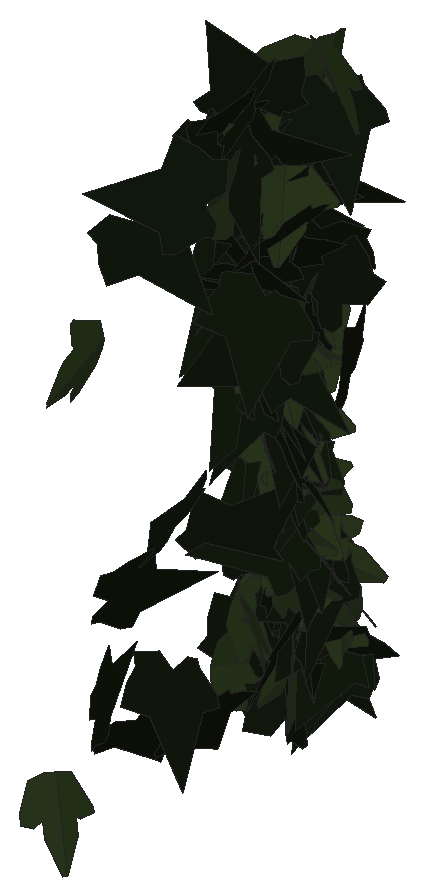
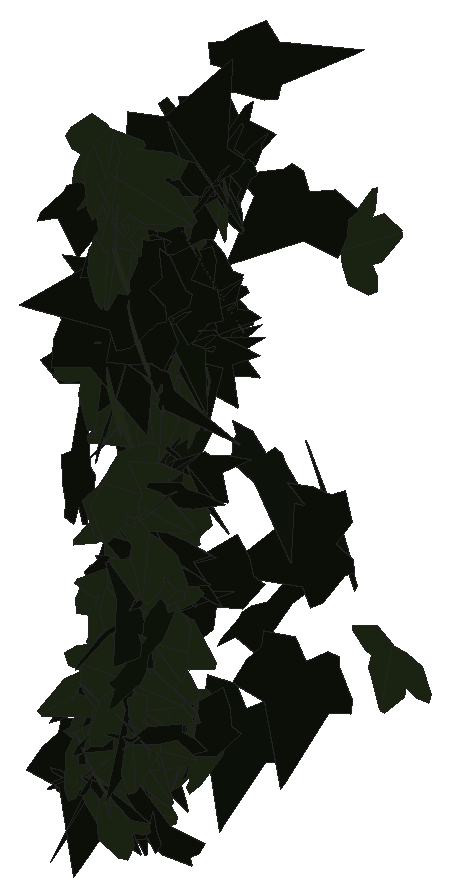
# SketchUp Ruby script. Lengths in inches.
U = 1.inch
M = Sketchup.active_model
def pt(a) = Geom::Point3d.new(a.map { |v| v * U })
def face(e, loops, mat)
  f = e.add_face(loops[0].map { |a| pt(a) })
  loops[1..].each { |l| e.add_face(l.map { |a| pt(a) }).erase! }
  f.material = f.back_material = mat if mat
  f
end
# faces: each face lists its corners as indices into pts; further lists are holes
def faces(e, pts, list, mat = nil) = list.each { |f| face(e, (f[0].is_a?(Array) ? f : [f]).map { |l| l.map { |i| pts[i] } }, mat) }
# xy, xz, yz: faces in a plane at the given z, y or x. An outline is a flat list of corners, or four numbers for a rectangle; further outlines are holes
def ring(l) = l.size == 4 ? [[l[0], l[1]], [l[2], l[1]], [l[2], l[3]], [l[0], l[3]]] : l.each_slice(2).to_a
def flat(e, list, mat, &to3) = list.each { |f| face(e, (f[0].is_a?(Array) ? f : [f]).map { |l| ring(l).map { |u, v| to3.(u, v) } }, mat) }
def xy(e, z, list, mat = nil) = flat(e, list, mat) { |x, y| [x, y, z] }
def xz(e, y, list, mat = nil) = flat(e, list, mat) { |x, z| [x, y, z] }
def yz(e, x, list, mat = nil) = flat(e, list, mat) { |y, z| [x, y, z] }
def lines(e, pts, list) = list.each { |a, b| e.add_line(pt(pts[a]), pt(pts[b])) }
# prism: a flat outline (further loops are holes) pulled along v
def prism(e, loops, v, mat = nil)
  f = face(e, loops, mat); d = Geom::Vector3d.new(v.map { |x| x * U })
  f.pushpull(f.normal.samedirection?(d) ? d.length : -d.length)
end
def box(e, o, s, mat = nil) = prism(e, [[o, [o[0] + s[0], o[1], o[2]], [o[0] + s[0], o[1] + s[1], o[2]], [o[0], o[1] + s[1], o[2]]]], [0, 0, s[2]], mat)
def at(x, y, z, deg = 0) = Geom::Transformation.translation(pt([x, y, z])) * Geom::Transformation.rotation(ORIGIN, Z_AXIS, deg.degrees)
def axes(o, x, y, z) = Geom::Transformation.new([*x, 0, *y, 0, *z, 0, *pt(o).to_a, 1])
def part(name) = M.definitions.add(name)
# library, detail: a bought-in or finely detailed component or shape, given as its bounding box
def library(name, o, s) = part(name).tap { |d| box(d.entities, o, s) }
def detail(e, o, s) = box(e.add_group.entities, o, s)
def put(e, d, t, mat = nil) = e.add_instance(d, t).tap { |i| i.material = mat if mat }
def group(e, t, mat = nil) = e.add_group.tap { |g| g.transformation = t; g.material = mat if mat }.entities
root = M.entities
M.materials.add("efeu1").color = [18, 25, 13]
M.materials.add("efeu2").color = [43, 57, 29]
c1 = part("ivyleaf_10")
p = [[0,0.5,-0.03],[-0.0625,2.02,-0.43],[-0.19,2.01,-0.46],[-0.54,1.05,-0.29],[-0.52,0.625,-0.18],[-0.83,0.76,-0.28],
  [-1.16,0.64,-0.33],[-1.15,0.33,-0.24],[-0.77,-0.39,0.02],[-0.3,-0.51,0.16],[0.04,-0.48,0.23],[-0.02,2.01,-0.4375],
  [-0.06,2.01,-0.43],[0.04,-0.49,0.23],[0.67,-0.49,0.14],[1.38,0.36,-0.2],[1.375,0.51,-0.24],[0.81,0.65,-0.19],
  [0.62,0.59,-0.15],[0.6,1.09,-0.28],[0.5,1.23,-0.31]]
faces(c1.entities,p,[[0,1,2,3,4,5,6,7,8,9,10],[11,12,0,13,14,15,16,17,18,19,20]],"efeu2")
c2 = part("ivyleaf_9")
p = [[1.54,2.16,1.25],[1.36,2.04,1.19],[-0.21,0.99,0.68],[-0.71,1.11,0.82],[-0.85,0.86,0.67],[-0.8,0.17,0.21],
  [-0.9,-0.01,0.1],[-0.67,-0.16,-0.02],[-0.08,-0.08,-0.05],[-0.03,-0.6,-0.4],[0.65,-0.88,-0.66],[0.83,-0.6,-0.49],
  [1.29,-0.42,-0.43],[1.8125,-0.07,-0.26],[1.21,0.44,0.15]]
faces(c2.entities,p,[[0,1,2,3,4,5,6,7,8,9,10,11,12,13,14]],"efeu1")
put(root,c1,axes([53.47,219.33,214.4],[0.45704,-0.01412,0.20227],[0.20232,-0.00106,-0.45724],[0.01334,0.4998,0.00475]))
put(root,c2,axes([54,219.53,215.61],[-0.09301,0.33525,0.35911],[0.09611,-0.34601,0.34791],[0.48178,0.13374,-0.00008]))
put(root,c1,axes([53.34,220.18,220.24],[0.05439,-0.10599,0.4856],[0.16699,-0.4562,-0.11828],[0.46814,0.17505,-0.01423]))
put(root,c2,axes([54.5625,220.84,222.49],[-0.22978,-0.0549,0.44067],[-0.41817,-0.14023,-0.23552],[0.14945,-0.47678,0.01853]))
put(root,c2,axes([54.08,220.91,215.59],[0.02323,-0.49581,-0.06029],[-0.00815,0.05997,-0.49632],[0.49939,0.02404,-0.0053]))
put(root,c2,axes([53.34,220.66,216.53],[0.2112,0.19575,0.40875],[0.30889,0.26781,-0.28786],[-0.33163,0.37411,-0.00781]))
put(root,c2,axes([53.63,220.79,214.85],[0.15717,0.47438,-0.01634],[-0.00665,-0.01501,-0.49973],[-0.47461,0.1573,0.00159]))
put(root,c2,axes([53.98,221.06,217.62],[-0.15319,0.43734,0.18779],[-0.08974,0.1672,-0.46259],[-0.46742,-0.17543,0.02727]))
put(root,c2,axes([53.2,221.3,221.49],[-0.08116,-0.15363,-0.46884],[0.22372,0.41202,-0.17374],[0.43973,-0.23798,0.00186]))
put(root,c2,axes([53.83,221.66,214.54],[0.0958,0.48707,0.05985],[0.0154,0.05797,-0.49639],[-0.49049,0.09695,-0.00389]))
put(root,c2,axes([53.6,222.34,222.27],[0.05873,-0.13634,-0.47745],[0.3246,-0.35328,0.14081],[-0.37575,-0.3265,0.04702]))
put(root,c2,axes([54.29,222.45,221.14],[-0.33156,0.20634,-0.31223],[0.18957,-0.26708,-0.3778],[-0.32269,-0.36891,0.09888]))
put(root,c2,axes([53.94,222.71,219.47],[-0.13657,-0.25069,0.41049],[-0.18242,-0.36785,-0.28533],[0.44506,-0.22769,0.00901]))
put(root,c2,axes([54.14,222.63,220.18],[-0.22139,-0.43521,-0.10761],[0.07488,0.08244,-0.48744],[0.44202,-0.23194,0.02868]))
put(root,c2,axes([53.73,222.52,222.24],[-0.23742,-0.09868,-0.42883],[0.39803,0.15961,-0.2571],[0.18763,-0.46345,0.00277]))
put(root,c1,axes([53.88,222.09,221.6875],[0.06079,0.01229,0.49614],[-0.22717,0.4451,0.01681],[-0.44125,-0.22746,0.0597]))
put(root,c2,axes([53.34,222.49,222.29],[0.21797,-0.39358,-0.21814],[-0.10411,0.1917,-0.4499],[0.43778,0.24155,0.00162]))
put(root,c1,axes([53.55,222.63,222.17],[-0.37502,0.1499,-0.29477],[0.20132,-0.2501,-0.38331],[-0.26235,-0.40618,0.12723]))
put(root,c2,axes([53.55,223.05,220.01],[-0.32264,-0.36441,0.11448],[-0.03267,-0.12297,-0.48354],[0.38057,-0.3195,0.05554]))
put(root,c2,axes([53.42,222.8,220.5],[0.26216,-0.19668,0.37761],[0.32785,-0.18967,-0.32641],[0.27163,0.41874,0.02952]))
put(root,c2,axes([53.59,222.54,216.48],[-0.09428,-0.05385,0.48807],[0.4814,0.08782,0.10268],[-0.09679,0.48927,0.03528]))
put(root,c2,axes([53.51,222.32,222.43],[0.21033,0.24671,0.38065],[0.16327,0.35028,-0.31724],[-0.42321,0.25775,0.06679]))
put(root,c2,axes([53.9,222.69,222.86],[-0.35354,0.35307,-0.01877],[0.01329,-0.01326,-0.49965],[-0.35332,-0.35379,0]))
put(root,c2,axes([53.8125,222.64,220.5],[0.11834,0.44295,-0.19949],[-0.10328,-0.17769,-0.45581],[-0.47469,0.14909,0.04944]))
put(root,c1,axes([53.52,222.89,219.55],[-0.23828,0.28258,-0.33671],[0.22949,-0.24669,-0.36943],[-0.37491,-0.3306,-0.01214]))
put(root,c2,axes([53.5,223.01,220.34],[-0.10372,-0.4838,-0.07198],[0.01572,0.07024,-0.49479],[0.48887,-0.1049,0.00064]))
put(root,c2,axes([54.39,222.55,221.22],[0.03375,0.49552,0.05766],[-0.01993,0.05909,-0.4961],[-0.49846,0.03119,0.02374]))
put(root,c2,axes([53.62,222.96,221.45],[-0.44295,0.1099,-0.20424],[0.1989,-0.04646,-0.45638],[-0.11929,-0.48555,-0.00256]))
put(root,c2,axes([53.42,223.02,220.63],[0.05885,-0.4881,-0.09108],[0.02288,0.09429,-0.4905],[0.496,0.05356,0.03344]))
put(root,c2,axes([53.58,223.13,220.15],[-0.38781,-0.31167,-0.04966],[0.03391,0.03707,-0.49747],[0.31378,-0.38921,-0.00761]))
put(root,c2,axes([53.8,223.11,218.66],[-0.4671,0.01305,-0.17791],[0.17691,-0.02998,-0.46669],[-0.02285,-0.49893,0.02339]))
put(root,c1,axes([54.19,222.98,221.66],[0.28978,0.40413,-0.05207],[-0.03386,-0.03979,-0.49726],[-0.40606,0.29172,0.00431]))
put(root,c2,axes([53.56,223.29,217.78],[0.06969,-0.17383,0.4636],[0.15332,-0.43758,-0.18712],[0.47078,0.16824,-0.00769]))
put(root,c2,axes([54.12,223.34,216.48],[-0.29618,-0.10764,0.38818],[-0.30507,-0.25472,-0.3034],[0.26308,-0.41657,0.08521]))
put(root,c2,axes([54.16,222.85,219.15],[-0.47438,0.1547,0.03207],[0.02004,-0.04176,0.49785],[0.15671,0.47363,0.03342]))
put(root,c2,axes([53.6,223.17,222.54],[0.26503,0.10546,0.41065],[-0.41185,-0.05096,0.27889],[0.10068,-0.48609,0.05985]))
put(root,c2,axes([53.48,222.91,222],[0.27008,-0.00035,0.42078],[0.42073,0.00781,-0.27005],[-0.00638,0.49994,0.00451]))
put(root,c2,axes([54.07,222.95,219.33],[0.30816,-0.30373,-0.25056],[-0.07503,0.26705,-0.416],[0.38653,0.29399,0.11902]))
put(root,c1,axes([54.02,223.37,214.64],[-0.09182,0.20633,-0.44609],[0.15642,-0.41794,-0.22551],[-0.46594,-0.18097,0.0122]))
put(root,c2,axes([53.48,223.42,218.65],[-0.2953,-0.40096,0.04504],[0.01521,-0.06684,-0.49528],[0.40319,-0.29115,0.05167]))
put(root,c1,axes([53.5,222.73,214.73],[-0.02372,0.1363,0.48048],[-0.07574,0.47448,-0.13834],[-0.49366,-0.07935,-0.00186]))
put(root,c2,axes([53.83,223.33,217.62],[0.01448,-0.00098,0.49979],[0.2449,-0.43584,-0.00795],[0.43568,0.24503,-0.01214]))
put(root,c1,axes([53.95,223.0625,219.15],[0.40735,0.24659,0.15252],[0.10752,0.1158,-0.47437],[-0.26927,0.41927,0.04131]))
put(root,c2,axes([53.79,223.22,218.59],[0.33112,-0.37195,0.04491],[0.03145,-0.03213,-0.49797],[0.37333,0.3326,0.00212]))
put(root,c1,axes([53.91,223.09,219.21],[0.47663,0.06535,0.13621],[0.11409,0.13979,-0.46631],[-0.09903,0.47559,0.11834]))
put(root,c1,axes([53.64,223.08,220.07],[-0.22078,0.44861,0.00311],[-0.00355,0.00172,-0.49998],[-0.4486,-0.22079,0.00243]))
put(root,c1,axes([53.85,223.1,219.72],[-0.02069,-0.46548,-0.1814],[-0.009,0.18187,-0.46566],[0.49949,-0.016,-0.0159]))
put(root,c2,axes([53.59,223.19,220.75],[0.34192,0.35436,0.08673],[-0.06353,-0.05922,0.4924],[0.35924,-0.34774,0.00452]))
put(root,c1,axes([53.48,222.88,222.16],[-0.05785,-0.07101,-0.49154],[0.2676,0.41242,-0.09108],[0.41838,-0.27361,-0.00972]))
put(root,c1,axes([53.52,223.11,215.36],[-0.39141,0.30174,0.07581],[-0.06203,0.0437,-0.49421],[-0.30488,-0.39628,0.00323]))
put(root,c1,axes([53.97,223.28,217.81],[0.4933,0.06307,-0.05176],[-0.05207,-0.00087,-0.49728],[-0.06281,0.49601,0.00571]))
put(root,c2,axes([53.71,223.08,220.75],[-0.20825,0.45121,0.05513],[-0.00999,0.05608,-0.49674],[-0.45446,-0.208,-0.01435]))
put(root,c2,axes([53.82,223.58,218.29],[-0.00935,-0.49417,0.07558],[-0.01528,-0.07527,-0.49407],[0.49968,-0.01155,-0.0137]))
put(root,c1,axes([53.79,223.01,219.11],[0.12164,-0.01465,0.48476],[0.22688,0.44343,-0.04353],[-0.42864,0.23055,0.11452]))
put(root,c1,axes([53.52,223.09,215.37],[-0.02719,0.44028,0.2354],[-0.01072,0.23518,-0.44111],[-0.49915,-0.02903,-0.00335]))
put(root,c2,axes([53.47,223.12,214.79],[-0.16113,-0.08895,0.46489],[0.41974,0.20013,0.18377],[-0.21877,0.44949,0.01018]))
put(root,c2,axes([54.05,223.43,215.28],[-0.27229,0.31633,-0.27531],[0.17829,-0.20979,-0.41737],[-0.37957,-0.32546,0.00145]))
put(root,c2,axes([53.95,223.25,217.97],[0.39999,-0.20776,-0.21644],[-0.19569,0.09275,-0.45067],[0.22741,0.44523,-0.00711]))
put(root,c1,axes([53.75,223.33,215.83],[-0.46901,0.03674,0.16936],[-0.17002,-0.00298,-0.47019],[-0.03354,-0.49864,0.01529]))
put(root,c1,axes([53.96,223.71,217.04],[-0.09442,-0.34082,0.35345],[0.08265,-0.36582,-0.33067],[0.484,-0.00402,0.12542]))
put(root,c2,axes([53.91,223.1,220.57],[0.33088,0.37219,0.04468],[0.00446,0.05568,-0.49687],[-0.37483,0.32921,0.03353]))
put(root,c2,axes([53.76,223.64,217.76],[-0.47605,-0.15276,-0.00653],[0.00646,0.00124,-0.49996],[0.15276,-0.47609,0.0008]))
put(root,c2,axes([54.04,223.82,221.79],[-0.02184,-0.10626,-0.48809],[0.1885,-0.45419,0.09044],[-0.46259,-0.18006,0.0599]))
put(root,c2,axes([53.79,223.67,217.68],[-0.40296,-0.29036,-0.05757],[0.04841,0.03128,-0.49667],[0.29203,-0.40584,0.0029]))
put(root,c1,axes([53.91,223.53,216.5625],[0.4134,0.24502,-0.13806],[-0.12504,-0.05974,-0.48041],[-0.25192,0.43173,0.01189]))
put(root,c2,axes([53.76,223.59,213.86],[-0.06694,0.17325,0.46422],[0.19852,-0.41982,0.18531],[0.45399,0.20913,-0.01259]))
put(root,c2,axes([53.26,223.55,218.81],[0.314,-0.38533,0.0541],[0.09573,0.00912,-0.49067],[0.37715,0.31849,0.0795]))
put(root,c2,axes([53.46,223.19,221.08],[0.0781,0.138,-0.47419],[0.16613,0.44477,0.15679],[0.46508,-0.18204,0.02362]))
put(root,c2,axes([53.96,223.81,216.3],[0.02001,-0.46268,0.18848],[0.05368,-0.18554,-0.46119],[0.49671,0.03869,0.04225]))
put(root,c1,axes([53.75,223.6,217.04],[0.24291,0.34652,0.2663],[-0.15055,-0.21968,0.42318],[0.41028,-0.28577,-0.00239]))
put(root,c2,axes([53.8,223.75,217.43],[-0.33401,-0.34396,-0.14188],[0.13652,0.06407,-0.47672],[0.34613,-0.35719,0.05111]))
put(root,c1,axes([53.49,223.46,216.34],[-0.00129,-0.06489,0.49577],[0.46553,0.18072,0.02487],[-0.18242,0.46166,0.05995]))
put(root,c1,axes([53.6,223.5,216.46],[-0.38706,-0.30517,-0.08401],[0.06762,0.04992,-0.49288],[0.30921,-0.39291,0.00262]))
put(root,c2,axes([53.89,223.64,219.86],[-0.43694,0.08429,0.22799],[-0.22302,0.04748,-0.44498],[-0.09666,-0.49055,-0.00389]))
put(root,c1,axes([53.99,223.6,221],[0.30226,-0.38995,-0.08109],[-0.05233,0.06203,-0.49337],[0.39484,0.30674,-0.00332]))
put(root,c1,axes([54.07,223.58,217.09],[-0.4293,-0.24454,0.07683],[-0.06707,-0.03747,-0.49406],[0.24739,-0.43451,-0.00063]))
put(root,c1,axes([53.96,223.63,218.04],[0.20228,0.45403,-0.05425],[-0.00769,-0.05593,-0.4968],[-0.45719,0.20182,-0.01565]))
put(root,c1,axes([53.68,223.68,215.62],[0.45745,0.1948,-0.05283],[-0.04901,-0.01976,-0.4972],[-0.1958,0.46007,0.00102]))
put(root,c1,axes([53.62,223.89,220.83],[0.24918,-0.35435,0.2497],[0.14397,-0.20402,-0.43319],[0.40888,0.28778,0.00036]))
put(root,c2,axes([53.88,223.89,216.71],[0.08142,-0.4927,0.02484],[0.00457,-0.02442,-0.49938],[0.49331,0.08154,0.00053]))
put(root,c2,axes([54.37,223.83,219.74],[0.04772,0.02256,0.49721],[-0.49708,-0.02318,0.04876],[0.02525,-0.49895,0.02022]))
put(root,c2,axes([53.93,224.09,219.37],[-0.01902,-0.11465,0.48631],[0.0133,-0.4866,-0.1142],[0.49946,0.00859,0.02156]))
put(root,c1,axes([53.97,223.84,219.82],[0.217,-0.44756,0.05099],[0.01887,-0.04752,-0.49738],[0.45006,0.21779,-0.00373]))
put(root,c2,axes([53.41,223.99,218.65],[-0.37258,-0.32539,-0.07284],[0.09743,-0.00178,-0.49041],[0.31889,-0.37963,0.06474]))
put(root,c2,axes([54.17,224.11,214.75],[-0.23354,-0.42315,0.12807],[0.06724,-0.17715,-0.46271],[0.43696,-0.1989,0.13965]))
put(root,c1,axes([53.2,223.58,218.39],[0.1673,0.11037,0.45807],[0.37027,0.26982,-0.20024],[-0.29139,0.40622,0.00855]))
put(root,c2,axes([53.83,224.15,215.03],[-0.176,-0.38646,0.26396],[0.03098,-0.29101,-0.4054],[0.46697,-0.12635,0.12638]))
put(root,c2,axes([53.74,223.59,213.79],[-0.47434,0.07747,0.13785],[0.13626,-0.02089,0.48062],[0.08022,0.49352,-0.0013]))
put(root,c1,axes([53.89,223.59,217.09],[0.1902,0.39099,0.24689],[0.11956,0.2163,-0.43465],[-0.44669,0.22438,-0.01121]))
put(root,c2,axes([53.89,223.71,216.26],[0.47262,-0.16139,-0.02422],[-0.02228,0.00969,-0.49941],[0.16167,0.47314,0.00197]))
put(root,c2,axes([54.13,223.77,220.65],[0.17111,0.31482,-0.34872],[-0.16789,-0.30565,-0.35832],[-0.43879,0.23972,0.00111]))
put(root,c1,axes([53.69,224.17,214.44],[-0.02126,-0.21802,0.44946],[0.03297,-0.4495,-0.21648],[0.49846,0.02044,0.03349]))
put(root,c1,axes([54.09,223.88,220.06],[-0.46112,-0.17205,-0.08816],[0.13862,-0.13535,-0.46094],[0.13475,-0.44953,0.17252]))
put(root,c1,axes([54.01,223.87,215.07],[0.47403,0.14284,0.06994],[0.06483,0.02725,-0.49503],[-0.14524,0.47839,0.00731]))
put(root,c2,axes([53.71,223.96,215.55],[0.02749,-0.46616,-0.17873],[-0.01944,0.17786,-0.46689],[0.49887,0.03262,-0.00834]))
put(root,c2,axes([53.3,223.82,220.96],[0.3444,0.14634,-0.33162],[0.27851,0.18594,0.37129],[0.23199,-0.44047,0.04656]))
put(root,c2,axes([53.96,224.11,215.66],[-0.33255,-0.18396,-0.32491],[0.35593,-0.02477,-0.35028],[0.11278,-0.46427,0.14743]))
put(root,c1,axes([53.62,224.08,222.74],[0.23023,0.25014,-0.36664],[-0.30328,-0.21291,-0.33569],[-0.32406,0.37696,0.05369]))
put(root,c2,axes([54.14,224.03,222.45],[-0.06025,-0.46037,-0.18556],[0.02293,0.18414,-0.46429],[0.49583,-0.06445,-0.00107]))
put(root,c1,axes([53.65,224.21,221.91],[0.1259,-0.11619,0.46973],[0.36726,-0.2931,-0.17093],[0.31508,0.38806,0.01154]))
put(root,c2,axes([53.61,223.83,215.69],[-0.08513,-0.15935,-0.46622],[0.20959,0.41647,-0.18062],[0.4459,-0.22619,-0.00411]))
put(root,c2,axes([53.72,223.78,217.08],[0.32727,-0.20255,-0.31916],[-0.22006,0.24117,-0.3787],[0.30736,0.38834,0.06871]))
put(root,c1,axes([53.99,223.89,215.4],[-0.49385,0.05823,0.05217],[-0.05199,0.00456,-0.49727],[-0.05839,-0.49658,0.00155]))
put(root,c2,axes([53.63,223.65,215.79],[0.04009,-0.04346,-0.49649],[-0.35049,0.35166,-0.05908],[0.35433,0.35277,-0.00227]))
put(root,c1,axes([53.81,224,215.33],[-0.32216,0.00045,0.38238],[-0.37171,-0.11764,-0.31303],[0.08969,-0.48596,0.07613]))
put(root,c2,axes([54.05,223.83,214.84],[0.26841,-0.24831,-0.34102],[-0.21332,0.26882,-0.36364],[0.36394,0.3407,0.03837]))
put(root,c2,axes([53.31,224.14,216.58],[0.28842,-0.37391,0.16433],[0.11115,-0.12173,-0.47205],[0.39302,0.30882,0.0129]))
put(root,c2,axes([54.17,224.21,214.57],[-0.45446,-0.14732,-0.14751],[0.15384,0.00178,-0.47574],[0.14069,-0.4778,0.04371]))
put(root,c2,axes([53.58,223.83,221.21],[0.36435,0.04864,0.33894],[0.33609,0.04385,-0.36759],[-0.06548,0.49569,-0.00074]))
put(root,c2,axes([53.43,224.2,215.43],[-0.21275,-0.42272,-0.16138],[0.09,0.13523,-0.47288],[0.44344,-0.23026,0.01855]))
put(root,c1,axes([54.07,224.01,222.99],[-0.41773,0.23003,-0.15028],[0.13552,-0.0654,-0.47682],[-0.23902,-0.4391,-0.00771]))
put(root,c1,axes([53.875,224.31,214.76],[0.01679,-0.16418,-0.47198],[0.30649,-0.36961,0.13947],[-0.39469,-0.29399,0.08823]))
put(root,c2,axes([54.17,223.85,214.86],[0.3292,0.34769,-0.14402],[-0.10536,-0.09854,-0.47874],[-0.36128,0.34555,0.00839]))
put(root,c1,axes([53.23,224.125,218.07],[0.46052,-0.06605,0.1832],[0.18324,-0.01225,-0.46505],[0.06592,0.49547,0.01292]))
put(root,c1,axes([53.73,224.34,221.91],[0.03114,-0.39178,0.30909],[0.11748,-0.29523,-0.38605],[0.485,0.09667,0.07367]))
put(root,c1,axes([53.87,224.22,222.95],[0.05494,-0.4794,0.13099],[0.0367,-0.12752,-0.48207],[0.49562,0.06259,0.02118]))
put(root,c1,axes([53.93,224.1,216.16],[0.10835,0.06209,-0.48416],[-0.48811,0.01604,-0.10718],[0.00223,0.49587,0.06409]))
put(root,c2,axes([53.8,223.68,216.83],[-0.02205,0.27078,0.41975],[-0.01351,0.41969,-0.27144],[-0.49933,-0.02331,-0.0112]))
put(root,c1,axes([53.68,224.33,215.41],[-0.06781,-0.09241,0.48668],[-0.30402,-0.38007,-0.11453],[0.39112,-0.31146,-0.00464]))
put(root,c1,axes([53.52,224.36,218.86],[0.07869,0.24429,-0.42911],[-0.25859,-0.34978,-0.24655],[-0.42064,0.26073,0.07129]))
put(root,c2,axes([54.16,224.31,218.43],[0.02272,0.2041,0.45588],[-0.06472,-0.4513,0.20527],[0.49527,-0.06834,0.00591]))
put(root,c1,axes([54.09,224.21,215.09],[-0.01631,-0.49515,0.06751],[0.03384,-0.06849,-0.49413],[0.49859,-0.01155,0.03575]))
put(root,c1,axes([53.89,223.9375,216.06],[-0.23222,-0.14412,-0.41869],[0.37823,0.18127,-0.27218],[0.23024,-0.44314,0.02483]))
put(root,c1,axes([53.79,223.95,222.08],[0.03701,-0.41224,-0.28052],[-0.00076,0.28124,-0.4134],[0.49863,0.03103,0.02019]))
put(root,c1,axes([53.6,224.29,218.72],[0.26568,0.15275,-0.39507],[-0.34311,-0.19585,-0.30646],[-0.24837,0.43395,0.00075]))
put(root,c1,axes([53.49,224.14,215.83],[-0.26173,-0.42583,-0.01279],[0.01326,0.00686,-0.49978],[0.42582,-0.26196,0.0077]))
